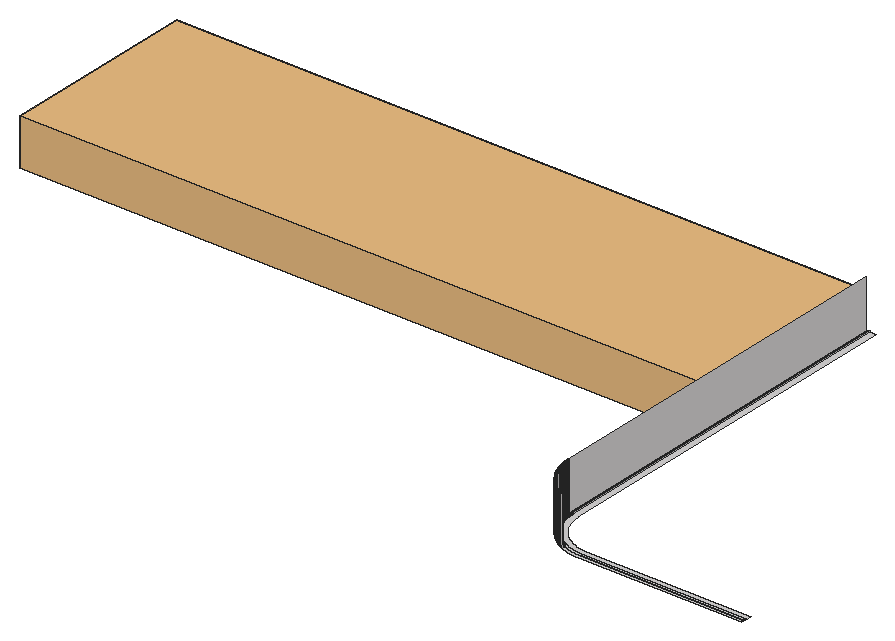
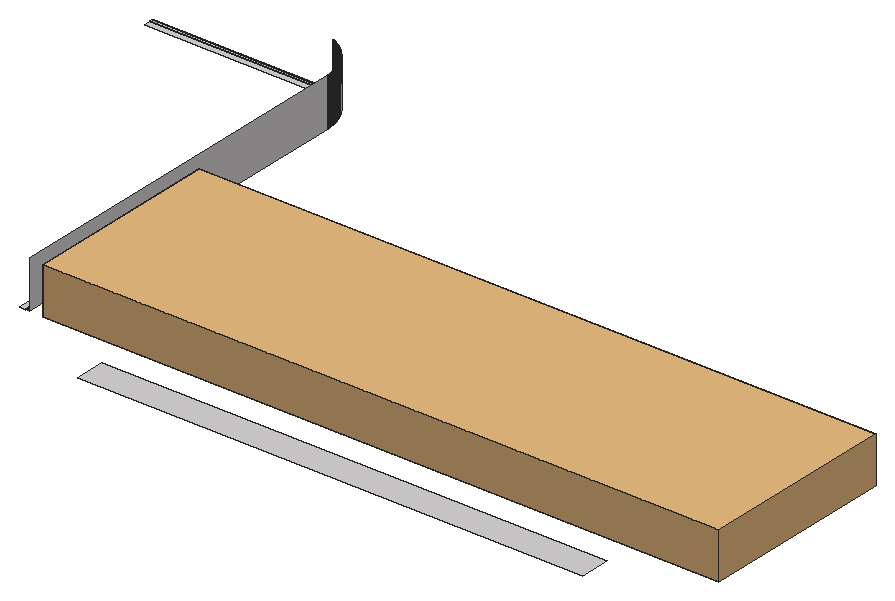
# SketchUp Ruby script. Lengths in inches.
U = 1.inch
M = Sketchup.active_model
def pt(a) = Geom::Point3d.new(a.map { |v| v * U })
def face(e, loops, mat)
  f = e.add_face(loops[0].map { |a| pt(a) })
  loops[1..].each { |l| e.add_face(l.map { |a| pt(a) }).erase! }
  f.material = f.back_material = mat if mat
  f
end
# faces: each face lists its corners as indices into pts; further lists are holes
def faces(e, pts, list, mat = nil) = list.each { |f| face(e, (f[0].is_a?(Array) ? f : [f]).map { |l| l.map { |i| pts[i] } }, mat) }
# xy, xz, yz: faces in a plane at the given z, y or x. An outline is a flat list of corners, or four numbers for a rectangle; further outlines are holes
def ring(l) = l.size == 4 ? [[l[0], l[1]], [l[2], l[1]], [l[2], l[3]], [l[0], l[3]]] : l.each_slice(2).to_a
def flat(e, list, mat, &to3) = list.each { |f| face(e, (f[0].is_a?(Array) ? f : [f]).map { |l| ring(l).map { |u, v| to3.(u, v) } }, mat) }
def xy(e, z, list, mat = nil) = flat(e, list, mat) { |x, y| [x, y, z] }
def xz(e, y, list, mat = nil) = flat(e, list, mat) { |x, z| [x, y, z] }
def yz(e, x, list, mat = nil) = flat(e, list, mat) { |y, z| [x, y, z] }
def lines(e, pts, list) = list.each { |a, b| e.add_line(pt(pts[a]), pt(pts[b])) }
# prism: a flat outline (further loops are holes) pulled along v
def prism(e, loops, v, mat = nil)
  f = face(e, loops, mat); d = Geom::Vector3d.new(v.map { |x| x * U })
  f.pushpull(f.normal.samedirection?(d) ? d.length : -d.length)
end
def box(e, o, s, mat = nil) = prism(e, [[o, [o[0] + s[0], o[1], o[2]], [o[0] + s[0], o[1] + s[1], o[2]], [o[0], o[1] + s[1], o[2]]]], [0, 0, s[2]], mat)
def at(x, y, z, deg = 0) = Geom::Transformation.translation(pt([x, y, z])) * Geom::Transformation.rotation(ORIGIN, Z_AXIS, deg.degrees)
def axes(o, x, y, z) = Geom::Transformation.new([*x, 0, *y, 0, *z, 0, *pt(o).to_a, 1])
def part(name) = M.definitions.add(name)
# library, detail: a bought-in or finely detailed component or shape, given as its bounding box
def library(name, o, s) = part(name).tap { |d| box(d.entities, o, s) }
def detail(e, o, s) = box(e.add_group.entities, o, s)
def put(e, d, t, mat = nil) = e.add_instance(d, t).tap { |i| i.material = mat if mat }
def group(e, t, mat = nil) = e.add_group.tap { |g| g.transformation = t; g.material = mat if mat }.entities
root = M.entities
M.materials.add("[Quartz Light Brown]").color = [215, 212, 212]
c1 = library("Group\#39",[0,0,-15.9],[195,66,15.9])
xy(root,348,[[33,266,180,275]],"[Quartz Light Brown]")
xy(root,354,[[215.8,143,215.61,143.01,215.41,143.01,215.21,143.02,215.02,143.03,214.82,143.05,214.63,143.0625,214.43,143.08,214.24,143.1,214.04,143.13,213.85,143.16,213.65,143.18,213.46,143.22,213.27,143.25,213.07,143.29,212.5,143.41,212.12,143.51,211.93,143.5625,211.74,143.62,211.55,143.67,211.36,143.73,211.18,143.8,210.99,143.86,210.81,143.93,210.44,144.07,210.26,144.14,209.54,144.46,209.37,144.55,209.19,144.63,209.02,144.73,208.84,144.82,208.67,144.91,208.16,145.21,208,145.3125,207.83,145.42,207.67,145.53,207.5,145.64,207.18,145.86,207.03,145.98,206.71,146.22,206.56,146.34,206.41,146.47,206.26,146.59,205.96,146.85,205.82,146.99,205.67,147.12,205.53,147.26,205.39,147.39,205.26,147.53,205.12,147.67,204.99,147.82,204.85,147.96,204.59,148.26,204.47,148.41,204.34,148.56,204.22,148.71,203.98,149.03,203.86,149.18,203.64,149.5,203.53,149.67,203.42,149.83,203.3125,150,203.21,150.16,202.91,150.67,202.82,150.84,202.73,151.02,202.63,151.19,202.55,151.37,202.46,151.54,202.14,152.26,202.07,152.44,201.93,152.81,201.86,152.99,201.8,153.18,201.73,153.36,201.67,153.55,201.62,153.74,201.5625,153.93,201.51,154.12,201.41,154.5,201.29,155.07,201.25,155.27,201.22,155.46,201.18,155.65,201.16,155.85,201.13,156.04,201.1,156.24,201.08,156.43,201.0625,156.63,201.05,156.82,201.03,157.02,201.02,157.21,201.01,157.41,201.01,157.61,201,157.8,201,266,201.75,266,201.75,157.625,201.76,157.44,201.77,157.25,201.78,157.07,201.79,156.88,201.81,156.7,201.83,156.51,201.85,156.33,201.87,156.14,201.9,155.96,201.93,155.77,201.96,155.59,201.99,155.4,202.02,155.22,202.0625,155.04,202.1,154.86,202.14,154.67,202.1875,154.49,202.24,154.3125,202.29,154.13,202.39,153.77,202.45,153.6,202.57,153.24,202.63,153.07,202.7,152.89,202.76,152.72,202.83,152.55,202.91,152.375,202.98,152.2,203.06,152.03,203.14,151.87,203.3,151.53,203.39,151.36,203.57,151.04,203.75,150.71,203.85,150.55,203.95,150.4,204.15,150.08,204.26,149.93,204.36,149.78,204.58,149.47,204.69,149.33,204.93,149.03,205.04,148.89,205.16,148.75,205.29,148.6,205.41,148.46,205.54,148.33,205.66,148.19,205.79,148.06,205.92,147.92,206.06,147.79,206.19,147.66,206.33,147.54,206.46,147.41,206.6,147.29,206.75,147.16,206.89,147.04,207.03,146.93,207.33,146.69,207.47,146.58,207.78,146.36,207.93,146.26,208.08,146.15,208.4,145.95,208.55,145.85,208.71,145.75,209.04,145.57,209.36,145.39,209.53,145.3,209.87,145.14,210.03,145.06,210.2,144.98,210.375,144.91,210.55,144.83,210.72,144.76,210.89,144.7,211.07,144.63,211.24,144.57,211.6,144.45,211.77,144.39,212.13,144.29,212.3125,144.24,212.49,144.1875,212.67,144.14,212.86,144.1,213.04,144.0625,213.22,144.02,213.4,143.99,213.59,143.96,213.77,143.93,213.96,143.9,214.14,143.87,214.33,143.85,214.51,143.83,214.7,143.81,214.88,143.79,215.07,143.78,215.25,143.77,215.44,143.76,215.625,143.75,263.5,143.75,263.5,143],[215.64,144.25,214.92,144.29,214.74,144.31,214.5625,144.33,214.38,144.35,214.21,144.37,214.03,144.39,213.49,144.48,213.32,144.51,213.14,144.55,212.97,144.59,212.79,144.63,212.62,144.67,212.44,144.72,212.27,144.77,212.09,144.82,211.75,144.92,211.07,145.16,210.9,145.23,210.74,145.3,210.57,145.37,210.41,145.4375,210.24,145.51,209.6,145.83,209.4375,145.92,209.28,146,208.97,146.18,208.82,146.28,208.66,146.37,208.21,146.67,208.0625,146.77,207.92,146.875,207.77,146.98,207.49,147.2,207.35,147.3125,207.21,147.43,207.07,147.54,206.93,147.66,206.67,147.9,206.54,148.03,206.41,148.15,206.15,148.41,206.03,148.54,205.9,148.67,205.66,148.93,205.54,149.07,205.43,149.21,205.3125,149.35,205.2,149.49,204.98,149.77,204.875,149.92,204.77,150.0625,204.67,150.21,204.37,150.66,204.28,150.82,204.18,150.97,204,151.28,203.92,151.4375,203.83,151.6,203.51,152.24,203.4375,152.41,203.37,152.57,203.3,152.74,203.23,152.9,203.16,153.07,202.92,153.75,202.82,154.09,202.77,154.27,202.72,154.44,202.67,154.62,202.63,154.79,202.59,154.97,202.55,155.14,202.51,155.32,202.48,155.49,202.39,156.03,202.37,156.21,202.35,156.38,202.33,156.5625,202.31,156.74,202.29,156.92,202.25,157.64,202.25,266,204,266,204,157.6875,204.01,157.53,204.02,157.37,204.03,157.22,204.05,156.9,204.07,156.75,204.08,156.59,204.1,156.43,204.125,156.28,204.15,156.12,204.17,155.97,204.2,155.8125,204.23,155.66,204.26,155.51,204.3,155.35,204.33,155.2,204.37,155.05,204.41,154.89,204.49,154.59,204.64,154.14,204.6875,153.99,204.74,153.85,204.8,153.7,204.85,153.55,204.91,153.41,204.97,153.26,205.04,153.12,205.1,152.98,205.17,152.83,205.45,152.27,205.53,152.14,205.61,152,205.6875,151.86,205.77,151.73,205.85,151.6,205.9375,151.46,206.02,151.33,206.2,151.07,206.29,150.95,206.38,150.82,206.48,150.69,206.58,150.57,206.67,150.45,206.77,150.33,206.98,150.09,207.08,149.97,207.1875,149.85,207.3,149.74,207.4,149.625,207.51,149.51,207.625,149.4,207.74,149.3,207.85,149.1875,207.97,149.08,208.09,148.98,208.33,148.77,208.45,148.67,208.57,148.58,208.69,148.48,208.82,148.38,208.95,148.29,209.07,148.2,209.33,148.02,209.46,147.9375,209.6,147.85,209.73,147.77,209.86,147.6875,210,147.61,210.14,147.53,210.27,147.45,210.83,147.17,210.98,147.1,211.12,147.04,211.26,146.97,211.41,146.91,211.55,146.85,211.7,146.8,211.85,146.74,211.99,146.6875,212.14,146.64,212.59,146.49,212.89,146.41,213.05,146.37,213.2,146.33,213.35,146.3,213.51,146.26,213.66,146.23,213.8125,146.2,213.97,146.17,214.12,146.15,214.28,146.125,214.43,146.1,214.59,146.08,214.75,146.07,214.9,146.05,215.22,146.03,215.37,146.02,215.53,146.01,215.6875,146,263.5,146,263.5,144.25]],"[Quartz Light Brown]")
xy(root,354.25,[[215.625,143.75,215.44,143.76,215.25,143.77,215.07,143.78,214.88,143.79,214.7,143.81,214.51,143.83,214.33,143.85,214.14,143.87,213.96,143.9,213.77,143.93,213.59,143.96,213.4,143.99,213.22,144.02,213.04,144.0625,212.86,144.1,212.67,144.14,212.49,144.1875,212.3125,144.24,212.13,144.29,211.77,144.39,211.6,144.45,211.24,144.57,211.07,144.63,210.89,144.7,210.72,144.76,210.55,144.83,210.375,144.91,210.2,144.98,210.03,145.06,209.87,145.14,209.53,145.3,209.36,145.39,209.04,145.57,208.71,145.75,208.55,145.85,208.4,145.95,208.08,146.15,207.93,146.26,207.78,146.36,207.47,146.58,207.33,146.69,207.03,146.93,206.89,147.04,206.75,147.16,206.6,147.29,206.46,147.41,206.33,147.54,206.19,147.66,206.06,147.79,205.92,147.92,205.79,148.06,205.66,148.19,205.54,148.33,205.41,148.46,205.29,148.6,205.16,148.75,205.04,148.89,204.93,149.03,204.69,149.33,204.58,149.47,204.36,149.78,204.26,149.93,204.15,150.08,203.95,150.4,203.85,150.55,203.75,150.71,203.57,151.04,203.39,151.36,203.3,151.53,203.14,151.87,203.06,152.03,202.98,152.2,202.91,152.375,202.83,152.55,202.76,152.72,202.7,152.89,202.63,153.07,202.57,153.24,202.45,153.6,202.39,153.77,202.29,154.13,202.24,154.3125,202.1875,154.49,202.14,154.67,202.1,154.86,202.0625,155.04,202.02,155.22,201.99,155.4,201.96,155.59,201.93,155.77,201.9,155.96,201.87,156.14,201.85,156.33,201.83,156.51,201.81,156.7,201.79,156.88,201.78,157.07,201.77,157.25,201.76,157.44,201.75,157.625,201.75,266,202.25,266,202.25,157.64,202.29,156.92,202.31,156.74,202.33,156.5625,202.35,156.38,202.37,156.21,202.39,156.03,202.48,155.49,202.51,155.32,202.55,155.14,202.59,154.97,202.63,154.79,202.67,154.62,202.72,154.44,202.77,154.27,202.82,154.09,202.92,153.75,203.16,153.07,203.23,152.9,203.3,152.74,203.37,152.57,203.4375,152.41,203.51,152.24,203.83,151.6,203.92,151.4375,204,151.28,204.18,150.97,204.28,150.82,204.37,150.66,204.67,150.21,204.77,150.0625,204.875,149.92,204.98,149.77,205.2,149.49,205.3125,149.35,205.43,149.21,205.54,149.07,205.66,148.93,205.9,148.67,206.03,148.54,206.15,148.41,206.41,148.15,206.54,148.03,206.67,147.9,206.93,147.66,207.07,147.54,207.21,147.43,207.35,147.3125,207.49,147.2,207.77,146.98,207.92,146.875,208.0625,146.77,208.21,146.67,208.66,146.37,208.82,146.28,208.97,146.18,209.28,146,209.4375,145.92,209.6,145.83,210.24,145.51,210.41,145.4375,210.57,145.37,210.74,145.3,210.9,145.23,211.07,145.16,211.75,144.92,212.09,144.82,212.27,144.77,212.44,144.72,212.62,144.67,212.79,144.63,212.97,144.59,213.14,144.55,213.32,144.51,213.49,144.48,214.03,144.39,214.21,144.37,214.38,144.35,214.5625,144.33,214.74,144.31,214.92,144.29,215.64,144.25,263.5,144.25,263.5,143.75]],"[Quartz Light Brown]")
yz(root,201,[[157.8,354,158,368],[158,354,266,368]],"[Quartz Light Brown]")
yz(root,201.01,[[157.41,354,157.61,368]],"[Quartz Light Brown]")
yz(root,201.75,[[157.625,354,157.8125,354.25],[157.8125,354,158,354.25],[158,354,266,354.25]],"[Quartz Light Brown]")
yz(root,202.25,[[157.64,354,157.82,354.25],[157.82,354,158,354.25],[158,354,266,354.25]],"[Quartz Light Brown]")
p = [[210.08,144.22,368],[210.08,144.22,354],[210.26,144.14,354],[210.26,144.14,368],[209.9,144.3,368],[209.9,144.3,354],
  [209.72,144.38,368],[209.72,144.38,354],[209.54,144.46,368],[209.54,144.46,354],[209.19,144.63,368],[209.19,144.63,354],
  [209.37,144.55,354],[209.37,144.55,368],[209.02,144.73,368],[209.02,144.73,354],[208.84,144.82,368],[208.84,144.82,354],
  [208.67,144.91,368],[208.67,144.91,354],[208.5,145.01,368],[208.5,145.01,354],[208.33,145.11,368],[208.33,145.11,354],
  [210.2,144.98,354],[210.03,145.06,354],[210.03,145.06,354.25],[210.2,144.98,354.25],[208.16,145.21,368],[208.16,145.21,354],
  [209.87,145.14,354],[209.7,145.22,354],[209.7,145.22,354.25],[209.87,145.14,354.25],[208,145.3125,368],[208,145.3125,354],
  [209.53,145.3,354],[209.53,145.3,354.25],[207.83,145.42,368],[207.83,145.42,354],[209.36,145.39,354],[209.36,145.39,354.25],
  [207.67,145.53,368],[207.67,145.53,354],[209.2,145.48,354],[209.2,145.48,354.25],[207.5,145.64,368],[207.5,145.64,354],
  [209.04,145.57,354],[209.04,145.57,354.25],[210.08,145.59,354],[210.24,145.51,354],[210.24,145.51,354.25],[210.08,145.59,354.25],
  [207.34,145.75,368],[207.34,145.75,354],[208.875,145.66,354],[208.875,145.66,354.25],[209.92,145.67,354],[209.92,145.67,354.25],
  [208.71,145.75,354],[208.71,145.75,354.25],[209.6,145.83,354],[209.76,145.75,354],[209.76,145.75,354.25],[209.6,145.83,354.25],
  [207.18,145.86,368],[207.18,145.86,354],[208.55,145.85,354],[208.4,145.95,354],[208.4,145.95,354.25],[208.55,145.85,354.25],
  [209.4375,145.92,354],[209.4375,145.92,354.25],[207.03,145.98,368],[207.03,145.98,354],[208.24,146.05,354],[208.24,146.05,354.25],
  [209.28,146,354],[209.28,146,354.25],[206.87,146.1,368],[206.87,146.1,354],[208.08,146.15,354],[208.08,146.15,354.25],
  [209.125,146.09,354],[209.125,146.09,354.25],[206.71,146.22,368],[206.71,146.22,354],[208.97,146.18,354],[208.97,146.18,354.25],
  [206.56,146.34,368],[206.56,146.34,354],[207.93,146.26,354],[207.93,146.26,354.25],[208.82,146.28,354],[208.82,146.28,354.25],
  [206.41,146.47,368],[206.41,146.47,354],[207.78,146.36,354],[207.78,146.36,354.25],[208.66,146.37,354],[208.66,146.37,354.25],
  [207.625,146.47,354],[207.625,146.47,354.25],[208.51,146.47,354],[208.51,146.47,354.25],[206.26,146.59,368],[206.26,146.59,354],
  [207.47,146.58,354],[207.47,146.58,354.25],[208.36,146.57,354],[208.36,146.57,354.25],[206.11,146.72,368],[206.11,146.72,354],
  [207.33,146.69,354],[207.33,146.69,354.25],[208.21,146.67,354],[208.21,146.67,354.25],[205.96,146.85,368],[205.96,146.85,354],
  [207.18,146.81,354],[207.18,146.81,354.25],[208.0625,146.77,354],[208.0625,146.77,354.25],[207.03,146.93,354],[207.03,146.93,354.25],
  [207.92,146.875,354],[207.92,146.875,354.25],[205.82,146.99,368],[205.82,146.99,354],[206.89,147.04,354],[206.89,147.04,354.25],
  [207.77,146.98,354],[207.77,146.98,354.25],[205.67,147.12,368],[205.67,147.12,354],[206.75,147.16,354],[206.75,147.16,354.25],
  [207.63,147.09,354],[207.63,147.09,354.25],[205.53,147.26,368],[205.53,147.26,354],[207.49,147.2,354],[207.49,147.2,354.25],
  [206.6,147.29,354],[206.6,147.29,354.25],[207.35,147.3125,354],[207.35,147.3125,354.25],[205.39,147.39,368],[205.39,147.39,354],
  [206.46,147.41,354],[206.46,147.41,354.25],[207.21,147.43,354],[207.21,147.43,354.25],[205.26,147.53,368],[205.26,147.53,354],
  [206.33,147.54,354],[206.33,147.54,354.25],[207.07,147.54,354],[207.07,147.54,354.25],[205.12,147.67,368],[205.12,147.67,354],
  [206.19,147.66,354],[206.19,147.66,354.25],[206.93,147.66,354],[206.93,147.66,354.25],[204.99,147.82,368],[204.99,147.82,354],
  [206.06,147.79,354],[206.06,147.79,354.25],[206.8,147.78,354],[206.8,147.78,354.25],[204.85,147.96,368],[204.85,147.96,354],
  [205.92,147.92,354],[205.92,147.92,354.25],[206.67,147.9,354],[206.67,147.9,354.25],[205.79,148.06,354],[205.79,148.06,354.25],
  [206.54,148.03,354],[206.54,148.03,354.25],[204.72,148.11,368],[204.72,148.11,354],[206.41,148.15,354],[206.41,148.15,354.25],
  [204.59,148.26,368],[204.59,148.26,354],[205.66,148.19,354],[205.66,148.19,354.25],[205.54,148.33,354],[205.54,148.33,354.25],
  [206.28,148.28,354],[206.28,148.28,354.25],[204.47,148.41,368],[204.47,148.41,354],[205.41,148.46,354],[205.41,148.46,354.25],
  [206.15,148.41,354],[206.15,148.41,354.25],[204.34,148.56,368],[204.34,148.56,354],[206.03,148.54,354],[206.03,148.54,354.25],
  [205.29,148.6,354],[205.29,148.6,354.25],[205.9,148.67,354],[205.9,148.67,354.25],[204.22,148.71,368],[204.22,148.71,354],
  [205.16,148.75,354],[205.16,148.75,354.25],[204.1,148.87,368],[204.1,148.87,354],[205.04,148.89,354],[205.04,148.89,354.25],
  [205.78,148.8,354],[205.78,148.8,354.25],[205.66,148.93,354],[205.66,148.93,354.25],[203.98,149.03,368],[203.98,149.03,354],
  [204.93,149.03,354],[204.93,149.03,354.25],[205.54,149.07,354],[205.54,149.07,354.25],[203.86,149.18,368],[203.86,149.18,354],
  [204.81,149.18,354],[204.81,149.18,354.25],[205.43,149.21,354],[205.43,149.21,354.25],[203.75,149.34,368],[203.75,149.34,354],
  [204.69,149.33,354],[204.69,149.33,354.25],[205.3125,149.35,354],[205.3125,149.35,354.25],[203.64,149.5,368],[203.64,149.5,354],
  [204.58,149.47,354],[204.58,149.47,354.25],[205.2,149.49,354],[205.2,149.49,354.25],[203.53,149.67,368],[203.53,149.67,354],
  [204.47,149.625,354],[204.47,149.625,354.25],[205.09,149.63,354],[205.09,149.63,354.25],[204.36,149.78,354],[204.36,149.78,354.25],
  [204.98,149.77,354],[204.98,149.77,354.25],[203.42,149.83,368],[203.42,149.83,354],[203.3125,150,368],[203.3125,150,354],
  [204.26,149.93,354],[204.26,149.93,354.25],[204.875,149.92,354],[204.875,149.92,354.25],[204.15,150.08,354],[204.15,150.08,354.25],
  [204.77,150.0625,354],[204.77,150.0625,354.25],[203.21,150.16,368],[203.21,150.16,354],[204.05,150.24,354],[204.05,150.24,354.25],
  [204.67,150.21,354],[204.67,150.21,354.25],[203.11,150.33,368],[203.11,150.33,354],[203.95,150.4,354],[203.95,150.4,354.25],
  [204.57,150.36,354],[204.57,150.36,354.25],[203.01,150.5,368],[203.01,150.5,354],[203.85,150.55,354],[203.85,150.55,354.25],
  [204.47,150.51,354],[204.47,150.51,354.25],[202.91,150.67,368],[202.91,150.67,354],[204.37,150.66,354],[204.37,150.66,354.25],
  [203.75,150.71,354],[203.75,150.71,354.25],[202.82,150.84,368],[202.82,150.84,354],[203.66,150.875,354],[203.66,150.875,354.25],
  [204.28,150.82,354],[204.28,150.82,354.25],[202.73,151.02,368],[202.73,151.02,354],[204.18,150.97,354],[204.18,150.97,354.25],
  [203.57,151.04,354],[203.57,151.04,354.25],[202.63,151.19,368],[202.63,151.19,354],[203.48,151.2,354],[203.48,151.2,354.25],
  [204.09,151.125,354],[204.09,151.125,354.25],[204,151.28,354],[204,151.28,354.25],[202.55,151.37,368],[202.55,151.37,354],
  [203.39,151.36,354],[203.39,151.36,354.25],[203.92,151.4375,354],[203.92,151.4375,354.25],[202.46,151.54,368],[202.46,151.54,354],
  [203.3,151.53,354],[203.3,151.53,354.25],[203.83,151.6,354],[203.83,151.6,354.25],[202.38,151.72,368],[202.38,151.72,354],
  [203.22,151.7,354],[203.22,151.7,354.25],[203.75,151.76,354],[203.75,151.76,354.25],[202.3,151.9,368],[202.3,151.9,354],
  [203.14,151.87,354],[203.14,151.87,354.25],[203.67,151.92,354],[203.67,151.92,354.25],[202.22,152.08,368],[202.22,152.08,354],
  [203.06,152.03,354],[203.06,152.03,354.25],[203.59,152.08,354],[203.59,152.08,354.25],[202.98,152.2,354],[202.98,152.2,354.25],
  [202.14,152.26,368],[202.14,152.26,354],[203.51,152.24,354],[203.51,152.24,354.25],[202.91,152.375,354],[202.91,152.375,354.25],
  [203.4375,152.41,354],[203.4375,152.41,354.25],[202.07,152.44,368],[202.07,152.44,354],[202,152.625,368],[202,152.625,354],
  [202.83,152.55,354],[202.83,152.55,354.25],[203.37,152.57,354],[203.37,152.57,354.25],[202.76,152.72,354],[202.76,152.72,354.25],
  [201.93,152.81,368],[201.93,152.81,354],[203.3,152.74,354],[203.3,152.74,354.25],[202.7,152.89,354],[202.7,152.89,354.25],
  [203.23,152.9,354],[203.23,152.9,354.25],[201.86,152.99,368],[201.86,152.99,354],[202.63,153.07,354],[202.63,153.07,354.25],
  [203.16,153.07,354],[203.16,153.07,354.25],[201.8,153.18,368],[201.8,153.18,354],[202.57,153.24,354],[202.57,153.24,354.25],
  [203.1,153.24,354],[203.1,153.24,354.25],[201.73,153.36,368],[201.73,153.36,354],[202.51,153.42,354],[202.51,153.42,354.25],
  [203.04,153.41,354],[203.04,153.41,354.25],[201.67,153.55,368],[201.67,153.55,354],[202.45,153.6,354],[202.45,153.6,354.25],
  [202.98,153.58,354],[202.98,153.58,354.25],[201.62,153.74,368],[201.62,153.74,354],[202.39,153.77,354],[202.39,153.77,354.25],
  [202.92,153.75,354],[202.92,153.75,354.25],[201.5625,153.93,368],[201.5625,153.93,354],[202.34,153.95,354],[202.34,153.95,354.25],
  [202.87,153.92,354],[202.87,153.92,354.25],[201.51,154.12,368],[201.51,154.12,354],[202.82,154.09,354],[202.82,154.09,354.25],
  [202.29,154.13,354],[202.29,154.13,354.25],[201.46,154.31,368],[201.46,154.31,354],[202.24,154.3125,354],[202.24,154.3125,354.25],
  [202.77,154.27,354],[202.77,154.27,354.25],[201.41,154.5,368],[201.41,154.5,354],[202.1875,154.49,354],[202.1875,154.49,354.25],
  [202.72,154.44,354],[202.72,154.44,354.25],[202.67,154.62,354],[202.67,154.62,354.25],[201.37,154.69,368],[201.37,154.69,354],
  [202.14,154.67,354],[202.14,154.67,354.25],[202.63,154.79,354],[202.63,154.79,354.25],[201.33,154.88,368],[201.33,154.88,354],
  [202.1,154.86,354],[202.1,154.86,354.25],[202.59,154.97,354],[202.59,154.97,354.25],[201.29,155.07,368],[201.29,155.07,354],
  [202.0625,155.04,354],[202.0625,155.04,354.25],[202.02,155.22,354],[202.02,155.22,354.25],[202.55,155.14,354],[202.55,155.14,354.25],
  [201.25,155.27,368],[201.25,155.27,354],[202.51,155.32,354],[202.51,155.32,354.25],[201.99,155.4,354],[201.99,155.4,354.25],
  [201.22,155.46,368],[201.22,155.46,354],[202.48,155.49,354],[202.48,155.49,354.25],[201.96,155.59,354],[201.96,155.59,354.25],
  [201.18,155.65,368],[201.18,155.65,354],[202.45,155.67,354],[202.45,155.67,354.25],[201.93,155.77,354],[201.93,155.77,354.25],
  [201.16,155.85,368],[201.16,155.85,354],[202.42,155.85,354],[202.42,155.85,354.25],[201.13,156.04,368],[201.13,156.04,354],
  [201.9,155.96,354],[201.9,155.96,354.25],[202.39,156.03,354],[202.39,156.03,354.25],[201.1,156.24,368],[201.1,156.24,354],
  [201.87,156.14,354],[201.87,156.14,354.25],[202.37,156.21,354],[202.37,156.21,354.25],[201.85,156.33,354],[201.85,156.33,354.25],
  [201.08,156.43,368],[201.08,156.43,354],[202.35,156.38,354],[202.35,156.38,354.25],[201.83,156.51,354],[201.83,156.51,354.25],
  [201.0625,156.63,368],[201.0625,156.63,354],[202.33,156.5625,354],[202.33,156.5625,354.25],[201.81,156.7,354],[201.81,156.7,354.25],
  [201.05,156.82,368],[201.05,156.82,354],[202.31,156.74,354],[202.31,156.74,354.25],[201.79,156.88,354],[201.79,156.88,354.25],
  [202.29,156.92,354],[202.29,156.92,354.25],[201.03,157.02,368],[201.03,157.02,354],[201.78,157.07,354],[201.78,157.07,354.25],
  [202.28,157.1,354],[202.28,157.1,354.25],[201.02,157.21,368],[201.02,157.21,354],[201.77,157.25,354],[201.77,157.25,354.25],
  [202.27,157.28,354],[202.27,157.28,354.25],[201.01,157.41,368],[201.01,157.41,354],[201.76,157.44,354],[201.76,157.44,354.25],
  [202.26,157.46,354],[202.26,157.46,354.25],[201.75,157.625,354],[201.75,157.625,354.25],[202.25,157.64,354],[202.25,157.64,354.25],
  [201,157.8,368],[201,157.8,354],[201.01,157.61,354],[201.01,157.61,368]]
faces(root,p,[[0,1,2,3],[4,5,1,0],[6,7,5,4],[8,9,7,6],[10,11,12,13],[13,12,9,8],[14,15,11,10],[16,17,15,14],
  [18,19,17,16],[20,21,19,18],[22,23,21,20],[24,25,26,27],[28,29,23,22],[30,31,32,33],[25,30,33,26],[34,35,29,28],
  [31,36,37,32],[38,39,35,34],[36,40,41,37],[42,43,39,38],[40,44,45,41],[46,47,43,42],[44,48,49,45],[50,51,52,53],
  [54,55,47,46],[48,56,57,49],[58,50,53,59],[56,60,61,57],[62,63,64,65],[63,58,59,64],[66,67,55,54],[68,69,70,71],
  [60,68,71,61],[72,62,65,73],[74,75,67,66],[69,76,77,70],[78,72,73,79],[80,81,75,74],[76,82,83,77],[84,78,79,85],
  [86,87,81,80],[88,84,85,89],[90,91,87,86],[82,92,93,83],[94,88,89,95],[96,97,91,90],[92,98,99,93],[100,94,95,101],
  [98,102,103,99],[104,100,101,105],[106,107,97,96],[102,108,109,103],[110,104,105,111],[112,113,107,106],[108,114,115,109],[116,110,111,117],
  [118,119,113,112],[114,120,121,115],[122,116,117,123],[120,124,125,121],[126,122,123,127],[128,129,119,118],[124,130,131,125],[132,126,127,133],
  [134,135,129,128],[130,136,137,131],[138,132,133,139],[140,141,135,134],[142,138,139,143],[136,144,145,137],[146,142,143,147],[148,149,141,140],
  [144,150,151,145],[152,146,147,153],[154,155,149,148],[150,156,157,151],[158,152,153,159],[160,161,155,154],[156,162,163,157],[164,158,159,165],
  [166,167,161,160],[162,168,169,163],[170,164,165,171],[172,173,167,166],[168,174,175,169],[176,170,171,177],[174,178,179,175],[180,176,177,181],
  [182,183,173,172],[184,180,181,185],[186,187,183,182],[178,188,189,179],[188,190,191,189],[192,184,185,193],[194,195,187,186],[190,196,197,191],
  [198,192,193,199],[200,201,195,194],[202,198,199,203],[196,204,205,197],[206,202,203,207],[208,209,201,200],[204,210,211,205],[212,213,209,208],
  [210,214,215,211],[216,206,207,217],[218,216,217,219],[220,221,213,212],[214,222,223,215],[224,218,219,225],[226,227,221,220],[222,228,229,223],
  [230,224,225,231],[232,233,227,226],[228,234,235,229],[236,230,231,237],[238,239,233,232],[234,240,241,235],[242,236,237,243],[244,245,239,238],
  [240,246,247,241],[248,242,243,249],[246,250,251,247],[252,248,249,253],[254,255,245,244],[256,257,255,254],[250,258,259,251],[260,252,253,261],
  [258,262,263,259],[264,260,261,265],[266,267,257,256],[262,268,269,263],[270,264,265,271],[272,273,267,266],[268,274,275,269],[276,270,271,277],
  [278,279,273,272],[274,280,281,275],[282,276,277,283],[284,285,279,278],[286,282,283,287],[280,288,289,281],[290,291,285,284],[288,292,293,289],
  [294,286,287,295],[296,297,291,290],[298,294,295,299],[292,300,301,293],[302,303,297,296],[300,304,305,301],[306,298,299,307],[308,306,307,309],
  [310,311,303,302],[304,312,313,305],[314,308,309,315],[316,317,311,310],[312,318,319,313],[320,314,315,321],[322,323,317,316],[318,324,325,319],
  [326,320,321,327],[328,329,323,322],[324,330,331,325],[332,326,327,333],[334,335,329,328],[330,336,337,331],[338,332,333,339],[336,340,341,337],
  [342,343,335,334],[344,338,339,345],[340,346,347,341],[348,344,345,349],[350,351,343,342],[352,353,351,350],[346,354,355,347],[356,348,349,357],
  [354,358,359,355],[360,361,353,352],[362,356,357,363],[358,364,365,359],[366,362,363,367],[368,369,361,360],[364,370,371,365],[372,366,367,373],
  [374,375,369,368],[370,376,377,371],[378,372,373,379],[380,381,375,374],[376,382,383,377],[384,378,379,385],[386,387,381,380],[382,388,389,383],
  [390,384,385,391],[392,393,387,386],[388,394,395,389],[396,390,391,397],[398,399,393,392],[394,400,401,395],[402,396,397,403],[404,405,399,398],
  [406,402,403,407],[400,408,409,401],[410,411,405,404],[408,412,413,409],[414,406,407,415],[416,417,411,410],[412,418,419,413],[420,414,415,421],
  [422,420,421,423],[424,425,417,416],[418,426,427,419],[428,422,423,429],[430,431,425,424],[426,432,433,427],[434,428,429,435],[436,437,431,430],
  [432,438,439,433],[438,440,441,439],[442,434,435,443],[444,445,437,436],[446,442,443,447],[440,448,449,441],[450,451,445,444],[452,446,447,453],
  [448,454,455,449],[456,457,451,450],[458,452,453,459],[454,460,461,455],[462,463,457,456],[464,458,459,465],[466,467,463,462],[460,468,469,461],
  [470,464,465,471],[472,473,467,466],[468,474,475,469],[476,470,471,477],[474,478,479,475],[480,481,473,472],[482,476,477,483],[478,484,485,479],
  [486,487,481,480],[488,482,483,489],[484,490,491,485],[492,493,487,486],[494,488,489,495],[490,496,497,491],[498,494,495,499],[500,501,493,492],
  [496,502,503,497],[504,498,499,505],[506,507,501,500],[502,508,509,503],[510,504,505,511],[512,513,507,506],[508,514,515,509],[516,510,511,517],
  [514,518,519,515],[520,516,517,521],[522,523,524,525]],"[Quartz Light Brown]")
put(root,c1,axes([2,207,366],[1.01026,0,0],[0,0.86364,0],[0,0,0.85]),"[Quartz Light Brown]")
